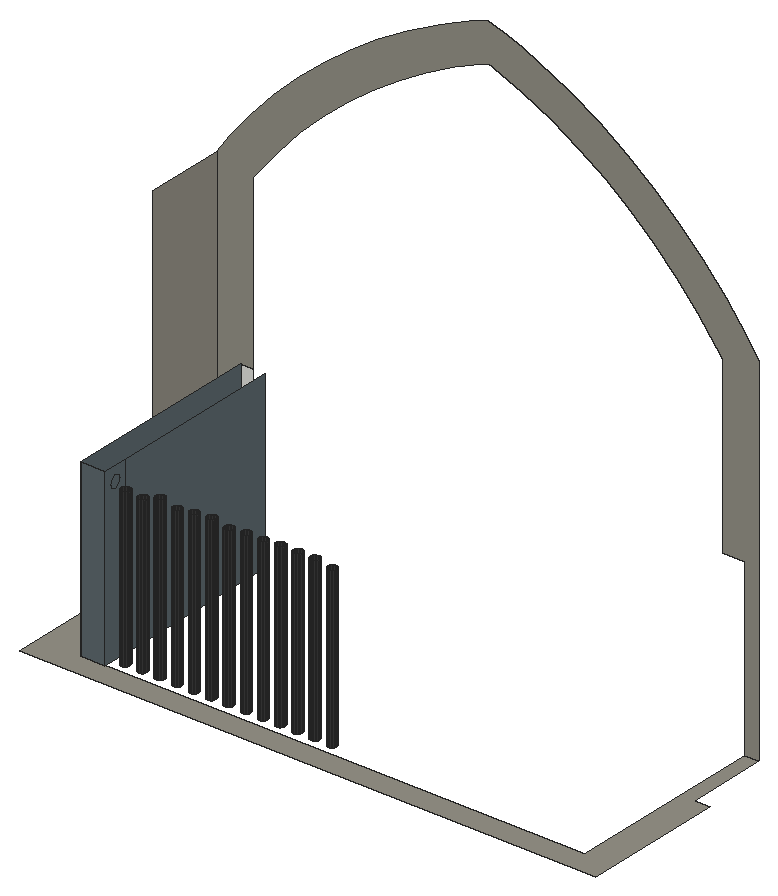
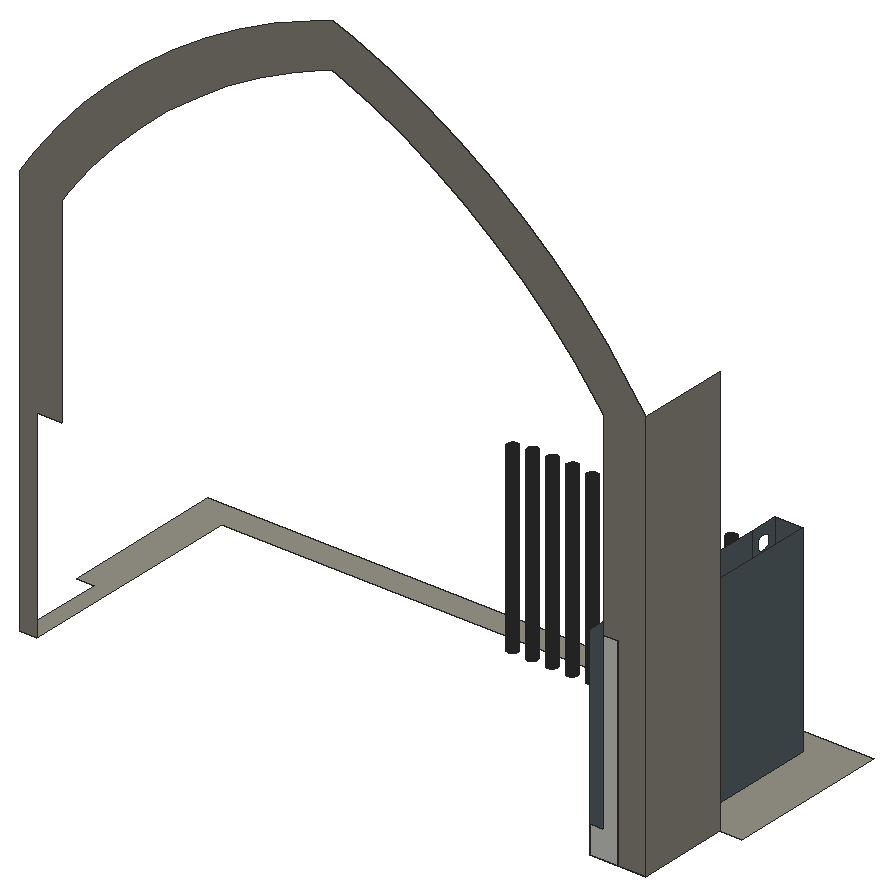
# SketchUp Ruby script. Lengths in inches.
U = 1.inch
M = Sketchup.active_model
def pt(a) = Geom::Point3d.new(a.map { |v| v * U })
def face(e, loops, mat)
  f = e.add_face(loops[0].map { |a| pt(a) })
  loops[1..].each { |l| e.add_face(l.map { |a| pt(a) }).erase! }
  f.material = f.back_material = mat if mat
  f
end
# faces: each face lists its corners as indices into pts; further lists are holes
def faces(e, pts, list, mat = nil) = list.each { |f| face(e, (f[0].is_a?(Array) ? f : [f]).map { |l| l.map { |i| pts[i] } }, mat) }
# xy, xz, yz: faces in a plane at the given z, y or x. An outline is a flat list of corners, or four numbers for a rectangle; further outlines are holes
def ring(l) = l.size == 4 ? [[l[0], l[1]], [l[2], l[1]], [l[2], l[3]], [l[0], l[3]]] : l.each_slice(2).to_a
def flat(e, list, mat, &to3) = list.each { |f| face(e, (f[0].is_a?(Array) ? f : [f]).map { |l| ring(l).map { |u, v| to3.(u, v) } }, mat) }
def xy(e, z, list, mat = nil) = flat(e, list, mat) { |x, y| [x, y, z] }
def xz(e, y, list, mat = nil) = flat(e, list, mat) { |x, z| [x, y, z] }
def yz(e, x, list, mat = nil) = flat(e, list, mat) { |y, z| [x, y, z] }
def lines(e, pts, list) = list.each { |a, b| e.add_line(pt(pts[a]), pt(pts[b])) }
# prism: a flat outline (further loops are holes) pulled along v
def prism(e, loops, v, mat = nil)
  f = face(e, loops, mat); d = Geom::Vector3d.new(v.map { |x| x * U })
  f.pushpull(f.normal.samedirection?(d) ? d.length : -d.length)
end
def box(e, o, s, mat = nil) = prism(e, [[o, [o[0] + s[0], o[1], o[2]], [o[0] + s[0], o[1] + s[1], o[2]], [o[0], o[1] + s[1], o[2]]]], [0, 0, s[2]], mat)
def at(x, y, z, deg = 0) = Geom::Transformation.translation(pt([x, y, z])) * Geom::Transformation.rotation(ORIGIN, Z_AXIS, deg.degrees)
def axes(o, x, y, z) = Geom::Transformation.new([*x, 0, *y, 0, *z, 0, *pt(o).to_a, 1])
def part(name) = M.definitions.add(name)
# library, detail: a bought-in or finely detailed component or shape, given as its bounding box
def library(name, o, s) = part(name).tap { |d| box(d.entities, o, s) }
def detail(e, o, s) = box(e.add_group.entities, o, s)
def put(e, d, t, mat = nil) = e.add_instance(d, t).tap { |i| i.material = mat if mat }
def group(e, t, mat = nil) = e.add_group.tap { |g| g.transformation = t; g.material = mat if mat }.entities
root = M.entities
M.materials.add("[Color M07]").color = [58, 58, 58]
M.materials.add("[Formica Graystone]").color = [149, 146, 135]
M.materials.add("[Formica Speckled Grey]").color = [94, 105, 111]
xy(root,557.29,[[223.35,116.47,226.66,144.04],[228.1,117.55,227.9375,117.57,227.79,117.63,227.66,117.73,227.56,117.86,227.5,118.01,227.48,118.17,227.5,118.33,227.56,118.48,227.66,118.61,227.79,118.71,227.9375,118.77,228.1,118.8,228.26,118.77,228.41,118.71,228.54,118.61,228.64,118.48,228.7,118.33,228.73,118.17,228.7,118.01,228.64,117.86,228.54,117.73,228.41,117.63,228.26,117.57],[230.48,117.55,230.3125,117.57,230.16,117.63,230.03,117.73,229.93,117.86,229.87,118.01,229.85,118.17,229.87,118.33,229.93,118.48,230.03,118.61,230.16,118.71,230.3125,118.77,230.48,118.8,230.64,118.77,230.79,118.71,230.92,118.61,231.02,118.48,231.08,118.33,231.1,118.17,231.08,118.01,231.02,117.86,230.92,117.73,230.79,117.63,230.64,117.57],[232.85,117.55,232.6875,117.57,232.54,117.63,232.41,117.73,232.31,117.86,232.25,118.01,232.23,118.17,232.25,118.33,232.31,118.48,232.41,118.61,232.54,118.71,232.6875,118.77,232.85,118.8,233.01,118.77,233.16,118.71,233.29,118.61,233.39,118.48,233.45,118.33,233.48,118.17,233.45,118.01,233.39,117.86,233.29,117.73,233.16,117.63,233.01,117.57],[235.23,117.55,235.0625,117.57,234.91,117.63,234.78,117.73,234.68,117.86,234.62,118.01,234.6,118.17,234.62,118.33,234.68,118.48,234.78,118.61,234.91,118.71,235.0625,118.77,235.23,118.8,235.39,118.77,235.54,118.71,235.67,118.61,235.77,118.48,235.83,118.33,235.85,118.17,235.83,118.01,235.77,117.86,235.67,117.73,235.54,117.63,235.39,117.57],
  [237.6,117.55,237.4375,117.57,237.29,117.63,237.16,117.73,237.06,117.86,237,118.01,236.98,118.17,237,118.33,237.06,118.48,237.16,118.61,237.29,118.71,237.4375,118.77,237.6,118.8,237.76,118.77,237.91,118.71,238.04,118.61,238.14,118.48,238.2,118.33,238.23,118.17,238.2,118.01,238.14,117.86,238.04,117.73,237.91,117.63,237.76,117.57],[239.98,117.55,239.8125,117.57,239.66,117.63,239.53,117.73,239.43,117.86,239.37,118.01,239.35,118.17,239.37,118.33,239.43,118.48,239.53,118.61,239.66,118.71,239.8125,118.77,239.98,118.8,240.14,118.77,240.29,118.71,240.42,118.61,240.52,118.48,240.58,118.33,240.6,118.17,240.58,118.01,240.52,117.86,240.42,117.73,240.29,117.63,240.14,117.57],[242.35,117.55,242.1875,117.57,242.04,117.63,241.91,117.73,241.81,117.86,241.75,118.01,241.73,118.17,241.75,118.33,241.81,118.48,241.91,118.61,242.04,118.71,242.1875,118.77,242.35,118.8,242.51,118.77,242.66,118.71,242.79,118.61,242.89,118.48,242.95,118.33,242.98,118.17,242.95,118.01,242.89,117.86,242.79,117.73,242.66,117.63,242.51,117.57],[244.73,117.55,244.5625,117.57,244.41,117.63,244.28,117.73,244.18,117.86,244.12,118.01,244.1,118.17,244.12,118.33,244.18,118.48,244.28,118.61,244.41,118.71,244.5625,118.77,244.73,118.8,244.89,118.77,245.04,118.71,245.17,118.61,245.27,118.48,245.33,118.33,245.35,118.17,245.33,118.01,245.27,117.86,245.17,117.73,245.04,117.63,244.89,117.57],[247.1,117.55,246.9375,117.57,246.79,117.63,246.66,117.73,246.56,117.86,246.5,118.01,246.48,118.17,246.5,118.33,246.56,118.48,246.66,118.61,246.79,118.71,246.9375,118.77,247.1,118.8,247.26,118.77,247.41,118.71,247.54,118.61,247.64,118.48,247.7,118.33,247.73,118.17,247.7,118.01,247.64,117.86,247.54,117.73,247.41,117.63,247.26,117.57],
  [249.48,117.55,249.3125,117.57,249.16,117.63,249.03,117.73,248.93,117.86,248.87,118.01,248.85,118.17,248.87,118.33,248.93,118.48,249.03,118.61,249.16,118.71,249.3125,118.77,249.48,118.8,249.64,118.77,249.79,118.71,249.92,118.61,250.02,118.48,250.08,118.33,250.1,118.17,250.08,118.01,250.02,117.86,249.92,117.73,249.79,117.63,249.64,117.57],[251.85,117.55,251.6875,117.57,251.54,117.63,251.41,117.73,251.31,117.86,251.25,118.01,251.23,118.17,251.25,118.33,251.31,118.48,251.41,118.61,251.54,118.71,251.6875,118.77,251.85,118.8,252.01,118.77,252.16,118.71,252.29,118.61,252.39,118.48,252.45,118.33,252.48,118.17,252.45,118.01,252.39,117.86,252.29,117.73,252.16,117.63,252.01,117.57],[254.23,117.55,254.0625,117.57,253.91,117.63,253.78,117.73,253.68,117.86,253.62,118.01,253.6,118.17,253.62,118.33,253.68,118.48,253.78,118.61,253.91,118.71,254.0625,118.77,254.23,118.8,254.39,118.77,254.54,118.71,254.67,118.61,254.77,118.48,254.83,118.33,254.85,118.17,254.83,118.01,254.77,117.86,254.67,117.73,254.54,117.63,254.39,117.57],[256.6,117.55,256.4375,117.57,256.29,117.63,256.16,117.73,256.06,117.86,256,118.01,255.98,118.17,256,118.33,256.06,118.48,256.16,118.61,256.29,118.71,256.4375,118.77,256.6,118.8,256.76,118.77,256.91,118.71,257.04,118.61,257.14,118.48,257.2,118.33,257.23,118.17,257.2,118.01,257.14,117.86,257.04,117.73,256.91,117.63,256.76,117.57]])
xy(root,557.29,[[217.39,113.35,296.83,113.35,296.83,132.97,294.7,132.97,294.7,144.04,292.74,144.04,292.74,116.47,223.35,116.47,223.35,144.04,220.02,144.04,220.02,132.97,217.39,132.97]],"[Formica Graystone]")
xz(root,116.47,[[223.35,557.29,226.66,581.29]],"[Formica Speckled Grey]")
xz(root,144.04,[[223.35,557.29,226.66,557.29,226.66,560.54,225.01,560.54,225.01,581.29,223.35,581.29]])
xz(root,144.04,[[220.02,557.29,223.35,557.29,223.35,581.29,225.01,581.29,225.01,604.82,225.75,605.875,228.5,609.35,231.45,612.66,234.59,615.78,237.91,618.71,241.4,621.4375,245.05,623.95,248.84,626.24,252.76,628.31,256.79,630.13,257.48,630.4,258.17,630.16,262.22,628.45,266.14,626.49,269.93,624.27,273.56,621.8125,277.03,619.12,280.31,616.21,283.39,613.09,286.27,609.77,288.92,606.28,289.71,605.08,289.71,581.29,292.74,581.29,292.74,557.29,294.7,557.29,294.7,606.58,293,609.17,290.15,612.92,287.06,616.49,283.75,619.84,280.22,622.97,276.5,625.86,272.59,628.5,268.52,630.88,264.31,632.99,262.125,633.92,259.96,634.83,257.4,635.71,254.87,634.75,252.55,633.7,250.5625,632.8,246.38,630.6,242.33,628.15,238.44,625.46,234.72,622.55,231.17,619.43,227.82,616.09,224.67,612.57,221.74,608.86,220.02,606.39]],"[Formica Graystone]")
yz(root,220.02,[[132.97,557.29,144.04,606.39]],"[Formica Graystone]")
yz(root,223.35,[[116.47,557.29,144.04,581.29]],"[Formica Speckled Grey]")
yz(root,226.66,[[[116.47,557.29,119.78,581.29],[118.19,578.44,117.96,578.47,117.75,578.56,117.57,578.7,117.43,578.88,117.34,579.09,117.31,579.32,117.34,579.54,117.43,579.76,117.57,579.9375,117.75,580.08,117.96,580.16,118.19,580.19,118.41,580.16,118.62,580.08,118.8,579.9375,118.94,579.76,119.03,579.54,119.06,579.32,119.03,579.09,118.94,578.88,118.8,578.7,118.62,578.56,118.41,578.47]],[119.78,557.29,144.04,581.29]],"[Formica Speckled Grey]")
p = [[227.9375,117.57,557.29],[228.1,117.55,557.29],[228.1,117.55,578.86],[227.9375,117.57,578.86],[227.9375,117.57,578.7],[228.26,117.57,557.29],
  [228.26,117.57,578.7],[228.26,117.57,578.86],[230.3125,117.57,557.29],[230.48,117.55,557.29],[230.48,117.55,578.67],[230.3125,117.57,578.67],
  [230.64,117.57,557.29],[230.64,117.57,578.67],[232.6875,117.57,557.29],[232.85,117.55,557.29],[232.85,117.55,579.54],[232.6875,117.57,579.54],
  [232.6875,117.57,578.7],[233.01,117.57,557.29],[233.01,117.57,578.7],[233.01,117.57,579.54],[235.0625,117.57,557.29],[235.23,117.55,557.29],
  [235.23,117.55,578.98],[235.0625,117.57,578.98],[235.0625,117.57,578.7],[235.39,117.57,557.29],[235.39,117.57,578.7],[235.39,117.57,578.98],
  [237.4375,117.57,557.29],[237.6,117.55,557.29],[237.6,117.55,579.32],[237.4375,117.57,579.32],[237.4375,117.57,578.7],[237.76,117.57,557.29],
  [237.76,117.57,578.7],[237.76,117.57,579.32],[239.8125,117.57,557.29],[239.98,117.55,557.29],[239.98,117.55,579.54],[239.8125,117.57,579.54],
  [239.8125,117.57,578.7],[240.14,117.57,557.29],[240.14,117.57,578.7],[240.14,117.57,579.54],[242.1875,117.57,557.29],[242.35,117.55,557.29],
  [242.35,117.55,579.09],[242.1875,117.57,579.09],[242.1875,117.57,578.7],[242.51,117.57,557.29],[242.51,117.57,578.7],[242.51,117.57,579.09],
  [244.5625,117.57,557.29],[244.73,117.55,557.29],[244.73,117.55,579.32],[244.5625,117.57,579.32],[244.5625,117.57,578.7],[244.89,117.57,557.29],
  [244.89,117.57,578.7],[244.89,117.57,579.32],[246.9375,117.57,557.29],[247.1,117.55,557.29],[247.1,117.55,579.32],[246.9375,117.57,579.32],
  [246.9375,117.57,578.7],[247.26,117.57,557.29],[247.26,117.57,578.7],[247.26,117.57,579.32],[249.3125,117.57,557.29],[249.48,117.55,557.29],
  [249.48,117.55,579.54],[249.3125,117.57,579.54],[249.3125,117.57,578.7],[249.64,117.57,557.29],[249.64,117.57,578.7],[249.64,117.57,579.54],
  [251.6875,117.57,557.29],[251.85,117.55,557.29],[251.85,117.55,579.54],[251.6875,117.57,579.54],[251.6875,117.57,578.7],[252.01,117.57,557.29],
  [252.01,117.57,578.7],[252.01,117.57,579.54],[254.0625,117.57,557.29],[254.23,117.55,557.29],[254.23,117.55,579.54],[254.0625,117.57,579.54],
  [254.0625,117.57,578.7],[254.39,117.57,557.29],[254.39,117.57,578.7],[254.39,117.57,579.54],[256.4375,117.57,557.29],[256.6,117.55,557.29],
  [256.6,117.55,579.17],[256.4375,117.57,579.17],[256.4375,117.57,578.7],[256.76,117.57,557.29],[256.76,117.57,578.7],[256.76,117.57,579.17],
  [227.66,117.73,557.29],[227.79,117.63,557.29],[227.79,117.63,578.86],[227.66,117.73,578.86],[228.41,117.63,557.29],[228.41,117.63,578.86],
  [228.54,117.73,557.29],[228.54,117.73,578.86],[230.03,117.73,557.29],[230.16,117.63,557.29],[230.16,117.63,578.67],[230.03,117.73,578.67],
  [230.79,117.63,557.29],[230.79,117.63,578.67],[230.92,117.73,557.29],[230.92,117.73,578.67],[232.41,117.73,557.29],[232.54,117.63,557.29],
  [232.54,117.63,579.54],[232.41,117.73,579.54],[233.16,117.63,557.29],[233.16,117.63,579.54],[233.29,117.73,557.29],[233.29,117.73,579.54],
  [234.78,117.73,557.29],[234.91,117.63,557.29],[234.91,117.63,578.98],[234.78,117.73,578.98],[235.54,117.63,557.29],[235.54,117.63,578.98],
  [235.67,117.73,557.29],[235.67,117.73,578.98],[237.16,117.73,557.29],[237.29,117.63,557.29],[237.29,117.63,579.32],[237.16,117.73,579.32],
  [237.91,117.63,557.29],[237.91,117.63,579.32],[238.04,117.73,557.29],[238.04,117.73,579.32],[239.53,117.73,557.29],[239.66,117.63,557.29],
  [239.66,117.63,579.54],[239.53,117.73,579.54],[240.29,117.63,557.29],[240.29,117.63,579.54],[240.42,117.73,557.29],[240.42,117.73,579.54],
  [241.91,117.73,557.29],[242.04,117.63,557.29],[242.04,117.63,579.09],[241.91,117.73,579.09],[242.66,117.63,557.29],[242.66,117.63,579.09],
  [242.79,117.73,557.29],[242.79,117.73,579.09],[244.28,117.73,557.29],[244.41,117.63,557.29],[244.41,117.63,579.32],[244.28,117.73,579.32],
  [245.04,117.63,557.29],[245.04,117.63,579.32],[245.17,117.73,557.29],[245.17,117.73,579.32],[246.66,117.73,557.29],[246.79,117.63,557.29],
  [246.79,117.63,579.32],[246.66,117.73,579.32],[247.41,117.63,557.29],[247.41,117.63,579.32],[247.54,117.73,557.29],[247.54,117.73,579.32],
  [249.03,117.73,557.29],[249.16,117.63,557.29],[249.16,117.63,579.54],[249.03,117.73,579.54],[249.79,117.63,557.29],[249.79,117.63,579.54],
  [249.92,117.73,557.29],[249.92,117.73,579.54],[251.41,117.73,557.29],[251.54,117.63,557.29],[251.54,117.63,579.54],[251.41,117.73,579.54],
  [252.16,117.63,557.29],[252.16,117.63,579.54],[252.29,117.73,557.29],[252.29,117.73,579.54],[253.78,117.73,557.29],[253.91,117.63,557.29],
  [253.91,117.63,579.54],[253.78,117.73,579.54],[254.54,117.63,557.29],[254.54,117.63,579.54],[254.67,117.73,557.29],[254.67,117.73,579.54],
  [256.16,117.73,557.29],[256.29,117.63,557.29],[256.29,117.63,579.17],[256.16,117.73,579.17],[256.91,117.63,557.29],[256.91,117.63,579.17],
  [257.04,117.73,557.29],[257.04,117.73,579.17],[227.56,117.86,557.29],[227.56,117.86,578.86],[228.64,117.86,557.29],[228.64,117.86,578.86],
  [229.93,117.86,557.29],[229.93,117.86,578.67],[231.02,117.86,557.29],[231.02,117.86,578.67],[232.31,117.86,557.29],[232.31,117.86,579.54],
  [233.39,117.86,557.29],[233.39,117.86,579.54],[234.68,117.86,557.29],[234.68,117.86,578.98],[235.77,117.86,557.29],[235.77,117.86,578.98],
  [237.06,117.86,557.29],[237.06,117.86,579.32],[238.14,117.86,557.29],[238.14,117.86,579.32],[239.43,117.86,557.29],[239.43,117.86,579.54],
  [240.52,117.86,557.29],[240.52,117.86,579.54],[241.81,117.86,557.29],[241.81,117.86,579.09],[242.89,117.86,557.29],[242.89,117.86,579.09],
  [244.18,117.86,557.29],[244.18,117.86,579.32],[245.27,117.86,557.29],[245.27,117.86,579.32],[246.56,117.86,557.29],[246.56,117.86,579.32],
  [247.64,117.86,557.29],[247.64,117.86,579.32],[248.93,117.86,557.29],[248.93,117.86,579.54],[250.02,117.86,557.29],[250.02,117.86,579.54],
  [251.31,117.86,557.29],[251.31,117.86,579.54],[252.39,117.86,557.29],[252.39,117.86,579.54],[253.68,117.86,557.29],[253.68,117.86,579.54],
  [254.77,117.86,557.29],[254.77,117.86,579.54],[256.06,117.86,557.29],[256.06,117.86,579.17],[257.14,117.86,557.29],[257.14,117.86,579.17],
  [227.5,118.01,557.29],[227.5,118.01,578.86],[228.7,118.01,557.29],[228.7,118.01,578.86],[229.87,118.01,557.29],[229.87,118.01,578.67],
  [231.08,118.01,557.29],[231.08,118.01,578.67],[232.25,118.01,557.29],[232.25,118.01,579.54],[233.45,118.01,557.29],[233.45,118.01,579.54],
  [234.62,118.01,557.29],[234.62,118.01,578.98],[235.83,118.01,557.29],[235.83,118.01,578.98],[237,118.01,557.29],[237,118.01,579.32],
  [238.2,118.01,557.29],[238.2,118.01,579.32],[239.37,118.01,557.29],[239.37,118.01,579.54],[240.58,118.01,557.29],[240.58,118.01,579.54],
  [241.75,118.01,557.29],[241.75,118.01,579.09],[242.95,118.01,557.29],[242.95,118.01,579.09],[244.12,118.01,557.29],[244.12,118.01,579.32],
  [245.33,118.01,557.29],[245.33,118.01,579.32],[246.5,118.01,557.29],[246.5,118.01,579.32],[247.7,118.01,557.29],[247.7,118.01,579.32],
  [248.87,118.01,557.29],[248.87,118.01,579.54],[250.08,118.01,557.29],[250.08,118.01,579.54],[251.25,118.01,557.29],[251.25,118.01,579.54],
  [252.45,118.01,557.29],[252.45,118.01,579.54],[253.62,118.01,557.29],[253.62,118.01,579.54],[254.83,118.01,557.29],[254.83,118.01,579.54],
  [256,118.01,557.29],[256,118.01,579.17],[257.2,118.01,557.29],[257.2,118.01,579.17],[227.48,118.17,557.29],[227.48,118.17,578.86],
  [228.73,118.17,557.29],[228.73,118.17,578.86],[229.85,118.17,557.29],[229.85,118.17,578.67],[231.1,118.17,557.29],[231.1,118.17,578.67],
  [232.23,118.17,557.29],[232.23,118.17,579.54],[233.48,118.17,557.29],[233.48,118.17,579.54],[234.6,118.17,557.29],[234.6,118.17,578.98],
  [235.85,118.17,557.29],[235.85,118.17,578.98],[236.98,118.17,557.29],[236.98,118.17,579.32],[238.23,118.17,557.29],[238.23,118.17,579.32],
  [239.35,118.17,557.29],[239.35,118.17,579.54],[240.6,118.17,557.29],[240.6,118.17,579.54],[241.73,118.17,557.29],[241.73,118.17,579.09],
  [242.98,118.17,557.29],[242.98,118.17,579.09],[244.1,118.17,557.29],[244.1,118.17,579.32],[245.35,118.17,557.29],[245.35,118.17,579.32],
  [246.48,118.17,557.29],[246.48,118.17,579.32],[247.73,118.17,557.29],[247.73,118.17,579.32],[248.85,118.17,557.29],[248.85,118.17,579.54],
  [250.1,118.17,557.29],[250.1,118.17,579.54],[251.23,118.17,557.29],[251.23,118.17,579.54],[252.48,118.17,557.29],[252.48,118.17,579.54],
  [253.6,118.17,557.29],[253.6,118.17,579.54],[254.85,118.17,557.29],[254.85,118.17,579.54],[255.98,118.17,557.29],[255.98,118.17,579.17],
  [257.23,118.17,557.29],[257.23,118.17,579.17],[227.5,118.33,557.29],[227.5,118.33,578.86],[228.7,118.33,557.29],[228.7,118.33,578.86],
  [229.87,118.33,557.29],[229.87,118.33,578.67],[231.08,118.33,557.29],[231.08,118.33,578.67],[232.25,118.33,557.29],[232.25,118.33,579.54],
  [233.45,118.33,557.29],[233.45,118.33,579.54],[234.62,118.33,557.29],[234.62,118.33,578.98],[235.83,118.33,557.29],[235.83,118.33,578.98],
  [237,118.33,557.29],[237,118.33,579.32],[238.2,118.33,557.29],[238.2,118.33,579.32],[239.37,118.33,557.29],[239.37,118.33,579.54],
  [240.58,118.33,557.29],[240.58,118.33,579.54],[241.75,118.33,557.29],[241.75,118.33,579.09],[242.95,118.33,557.29],[242.95,118.33,579.09],
  [244.12,118.33,557.29],[244.12,118.33,579.32],[245.33,118.33,557.29],[245.33,118.33,579.32],[246.5,118.33,557.29],[246.5,118.33,579.32],
  [247.7,118.33,557.29],[247.7,118.33,579.32],[248.87,118.33,557.29],[248.87,118.33,579.54],[250.08,118.33,557.29],[250.08,118.33,579.54],
  [251.25,118.33,557.29],[251.25,118.33,579.54],[252.45,118.33,557.29],[252.45,118.33,579.54],[253.62,118.33,557.29],[253.62,118.33,579.54],
  [254.83,118.33,557.29],[254.83,118.33,579.54],[256,118.33,557.29],[256,118.33,579.17],[257.2,118.33,557.29],[257.2,118.33,579.17],
  [227.56,118.48,557.29],[227.56,118.48,578.86],[228.64,118.48,557.29],[228.64,118.48,578.86],[229.93,118.48,557.29],[229.93,118.48,578.67],
  [231.02,118.48,557.29],[231.02,118.48,578.67],[232.31,118.48,557.29],[232.31,118.48,579.54],[233.39,118.48,557.29],[233.39,118.48,579.54],
  [234.68,118.48,557.29],[234.68,118.48,578.98],[235.77,118.48,557.29],[235.77,118.48,578.98],[237.06,118.48,557.29],[237.06,118.48,579.32],
  [238.14,118.48,557.29],[238.14,118.48,579.32],[239.43,118.48,557.29],[239.43,118.48,579.54],[240.52,118.48,557.29],[240.52,118.48,579.54],
  [241.81,118.48,557.29],[241.81,118.48,579.09],[242.89,118.48,557.29],[242.89,118.48,579.09],[244.18,118.48,557.29],[244.18,118.48,579.32],
  [245.27,118.48,557.29],[245.27,118.48,579.32],[246.56,118.48,557.29],[246.56,118.48,579.32],[247.64,118.48,557.29],[247.64,118.48,579.32],
  [248.93,118.48,557.29],[248.93,118.48,579.54],[250.02,118.48,557.29],[250.02,118.48,579.54],[251.31,118.48,557.29],[251.31,118.48,579.54],
  [252.39,118.48,557.29],[252.39,118.48,579.54],[253.68,118.48,557.29],[253.68,118.48,579.54],[254.77,118.48,557.29],[254.77,118.48,579.54],
  [256.06,118.48,557.29],[256.06,118.48,579.17],[257.14,118.48,557.29],[257.14,118.48,579.17],[227.66,118.61,557.29],[227.66,118.61,578.86],
  [228.54,118.61,557.29],[228.54,118.61,578.86],[230.03,118.61,557.29],[230.03,118.61,578.67],[230.92,118.61,557.29],[230.92,118.61,578.67],
  [232.41,118.61,557.29],[232.41,118.61,579.54],[233.29,118.61,557.29],[233.29,118.61,579.54],[234.78,118.61,557.29],[234.78,118.61,578.98],
  [235.67,118.61,557.29],[235.67,118.61,578.98],[237.16,118.61,557.29],[237.16,118.61,579.32],[238.04,118.61,557.29],[238.04,118.61,579.32],
  [239.53,118.61,557.29],[239.53,118.61,579.54],[240.42,118.61,557.29],[240.42,118.61,579.54],[241.91,118.61,557.29],[241.91,118.61,579.09],
  [242.79,118.61,557.29],[242.79,118.61,579.09],[244.28,118.61,557.29],[244.28,118.61,579.32],[245.17,118.61,557.29],[245.17,118.61,579.32],
  [246.66,118.61,557.29],[246.66,118.61,579.32],[247.54,118.61,557.29],[247.54,118.61,579.32],[249.03,118.61,557.29],[249.03,118.61,579.54],
  [249.92,118.61,557.29],[249.92,118.61,579.54],[251.41,118.61,557.29],[251.41,118.61,579.54],[252.29,118.61,557.29],[252.29,118.61,579.54],
  [253.78,118.61,557.29],[253.78,118.61,579.54],[254.67,118.61,557.29],[254.67,118.61,579.54],[256.16,118.61,557.29],[256.16,118.61,579.17],
  [257.04,118.61,557.29],[257.04,118.61,579.17],[227.79,118.71,557.29],[227.79,118.71,578.86],[228.41,118.71,557.29],[228.41,118.71,578.86],
  [230.16,118.71,557.29],[230.16,118.71,578.67],[230.79,118.71,557.29],[230.79,118.71,578.67],[232.54,118.71,557.29],[232.54,118.71,579.54],
  [233.16,118.71,557.29],[233.16,118.71,579.54],[234.91,118.71,557.29],[234.91,118.71,578.98],[235.54,118.71,557.29],[235.54,118.71,578.98],
  [237.29,118.71,557.29],[237.29,118.71,579.32],[237.91,118.71,557.29],[237.91,118.71,579.32],[239.66,118.71,557.29],[239.66,118.71,579.54],
  [240.29,118.71,557.29],[240.29,118.71,579.54],[242.04,118.71,557.29],[242.04,118.71,579.09],[242.66,118.71,557.29],[242.66,118.71,579.09],
  [244.41,118.71,557.29],[244.41,118.71,579.32],[245.04,118.71,557.29],[245.04,118.71,579.32],[246.79,118.71,557.29],[246.79,118.71,579.32],
  [247.41,118.71,557.29],[247.41,118.71,579.32],[249.16,118.71,557.29],[249.16,118.71,579.54],[249.79,118.71,557.29],[249.79,118.71,579.54],
  [251.54,118.71,557.29],[251.54,118.71,579.54],[252.16,118.71,557.29],[252.16,118.71,579.54],[253.91,118.71,557.29],[253.91,118.71,579.54],
  [254.54,118.71,557.29],[254.54,118.71,579.54],[256.29,118.71,557.29],[256.29,118.71,579.17],[256.91,118.71,557.29],[256.91,118.71,579.17],
  [227.9375,118.77,557.29],[227.9375,118.77,578.86],[228.26,118.77,557.29],[228.26,118.77,578.86],[230.3125,118.77,557.29],[230.3125,118.77,578.67],
  [230.64,118.77,557.29],[230.64,118.77,578.67],[232.6875,118.77,557.29],[232.6875,118.77,579.54],[233.01,118.77,557.29],[233.01,118.77,579.54],
  [235.0625,118.77,557.29],[235.0625,118.77,578.98],[235.39,118.77,557.29],[235.39,118.77,578.98],[237.4375,118.77,557.29],[237.4375,118.77,579.32],
  [237.76,118.77,557.29],[237.76,118.77,579.32],[239.8125,118.77,557.29],[239.8125,118.77,579.54],[240.14,118.77,557.29],[240.14,118.77,579.54],
  [242.1875,118.77,557.29],[242.1875,118.77,579.09],[242.51,118.77,557.29],[242.51,118.77,579.09],[244.5625,118.77,557.29],[244.5625,118.77,579.32],
  [244.89,118.77,557.29],[244.89,118.77,579.32],[246.9375,118.77,557.29],[246.9375,118.77,579.32],[247.26,118.77,557.29],[247.26,118.77,579.32],
  [249.3125,118.77,557.29],[249.3125,118.77,579.54],[249.64,118.77,557.29],[249.64,118.77,579.54],[251.6875,118.77,557.29],[251.6875,118.77,579.54],
  [252.01,118.77,557.29],[252.01,118.77,579.54],[254.0625,118.77,557.29],[254.0625,118.77,579.54],[254.39,118.77,557.29],[254.39,118.77,579.54],
  [256.4375,118.77,557.29],[256.4375,118.77,579.17],[256.76,118.77,557.29],[256.76,118.77,579.17],[228.1,118.8,557.29],[228.1,118.8,578.86],
  [230.48,118.8,557.29],[230.48,118.8,578.67],[232.85,118.8,557.29],[232.85,118.8,579.54],[235.23,118.8,557.29],[235.23,118.8,578.98],
  [237.6,118.8,557.29],[237.6,118.8,579.32],[239.98,118.8,557.29],[239.98,118.8,579.54],[242.35,118.8,557.29],[242.35,118.8,579.09],
  [244.73,118.8,557.29],[244.73,118.8,579.32],[247.1,118.8,557.29],[247.1,118.8,579.32],[249.48,118.8,557.29],[249.48,118.8,579.54],
  [251.85,118.8,557.29],[251.85,118.8,579.54],[254.23,118.8,557.29],[254.23,118.8,579.54],[256.6,118.8,557.29],[256.6,118.8,579.17]]
faces(root,p,[[0,1,2,3,4],[1,5,6,7,2],[8,9,10,11],[9,12,13,10],[14,15,16,17,18],[15,19,20,21,16],[22,23,24,25,26],[23,27,28,29,24],
  [30,31,32,33,34],[31,35,36,37,32],[38,39,40,41,42],[39,43,44,45,40],[46,47,48,49,50],[47,51,52,53,48],[54,55,56,57,58],[55,59,60,61,56],
  [62,63,64,65,66],[63,67,68,69,64],[70,71,72,73,74],[71,75,76,77,72],[78,79,80,81,82],[79,83,84,85,80],[86,87,88,89,90],[87,91,92,93,88],
  [94,95,96,97,98],[95,99,100,101,96],[102,103,104,105],[103,0,4,3,104],[5,106,107,7,6],[106,108,109,107],[110,111,112,113],[111,8,11,112],
  [12,114,115,13],[114,116,117,115],[118,119,120,121],[119,14,18,17,120],[19,122,123,21,20],[122,124,125,123],[126,127,128,129],[127,22,26,25,128],
  [27,130,131,29,28],[130,132,133,131],[134,135,136,137],[135,30,34,33,136],[35,138,139,37,36],[138,140,141,139],[142,143,144,145],[143,38,42,41,144],
  [43,146,147,45,44],[146,148,149,147],[150,151,152,153],[151,46,50,49,152],[51,154,155,53,52],[154,156,157,155],[158,159,160,161],[159,54,58,57,160],
  [59,162,163,61,60],[162,164,165,163],[166,167,168,169],[167,62,66,65,168],[67,170,171,69,68],[170,172,173,171],[174,175,176,177],[175,70,74,73,176],
  [75,178,179,77,76],[178,180,181,179],[182,183,184,185],[183,78,82,81,184],[83,186,187,85,84],[186,188,189,187],[190,191,192,193],[191,86,90,89,192],
  [91,194,195,93,92],[194,196,197,195],[198,199,200,201],[199,94,98,97,200],[99,202,203,101,100],[202,204,205,203],[206,102,105,207],[108,208,209,109],
  [210,110,113,211],[116,212,213,117],[214,118,121,215],[124,216,217,125],[218,126,129,219],[132,220,221,133],[222,134,137,223],[140,224,225,141],
  [226,142,145,227],[148,228,229,149],[230,150,153,231],[156,232,233,157],[234,158,161,235],[164,236,237,165],[238,166,169,239],[172,240,241,173],
  [242,174,177,243],[180,244,245,181],[246,182,185,247],[188,248,249,189],[250,190,193,251],[196,252,253,197],[254,198,201,255],[204,256,257,205],
  [258,206,207,259],[208,260,261,209],[262,210,211,263],[212,264,265,213],[266,214,215,267],[216,268,269,217],[270,218,219,271],[220,272,273,221],
  [274,222,223,275],[224,276,277,225],[278,226,227,279],[228,280,281,229],[282,230,231,283],[232,284,285,233],[286,234,235,287],[236,288,289,237],
  [290,238,239,291],[240,292,293,241],[294,242,243,295],[244,296,297,245],[298,246,247,299],[248,300,301,249],[302,250,251,303],[252,304,305,253],
  [306,254,255,307],[256,308,309,257],[310,258,259,311],[260,312,313,261],[314,262,263,315],[264,316,317,265],[318,266,267,319],[268,320,321,269],
  [322,270,271,323],[272,324,325,273],[326,274,275,327],[276,328,329,277],[330,278,279,331],[280,332,333,281],[334,282,283,335],[284,336,337,285],
  [338,286,287,339],[288,340,341,289],[342,290,291,343],[292,344,345,293],[346,294,295,347],[296,348,349,297],[350,298,299,351],[300,352,353,301],
  [354,302,303,355],[304,356,357,305],[358,306,307,359],[308,360,361,309],[362,310,311,363],[312,364,365,313],[366,314,315,367],[316,368,369,317],
  [370,318,319,371],[320,372,373,321],[374,322,323,375],[324,376,377,325],[378,326,327,379],[328,380,381,329],[382,330,331,383],[332,384,385,333],
  [386,334,335,387],[336,388,389,337],[390,338,339,391],[340,392,393,341],[394,342,343,395],[344,396,397,345],[398,346,347,399],[348,400,401,349],
  [402,350,351,403],[352,404,405,353],[406,354,355,407],[356,408,409,357],[410,358,359,411],[360,412,413,361],[414,362,363,415],[364,416,417,365],
  [418,366,367,419],[368,420,421,369],[422,370,371,423],[372,424,425,373],[426,374,375,427],[376,428,429,377],[430,378,379,431],[380,432,433,381],
  [434,382,383,435],[384,436,437,385],[438,386,387,439],[388,440,441,389],[442,390,391,443],[392,444,445,393],[446,394,395,447],[396,448,449,397],
  [450,398,399,451],[400,452,453,401],[454,402,403,455],[404,456,457,405],[458,406,407,459],[408,460,461,409],[462,410,411,463],[412,464,465,413],
  [466,414,415,467],[416,468,469,417],[470,418,419,471],[420,472,473,421],[474,422,423,475],[424,476,477,425],[478,426,427,479],[428,480,481,429],
  [482,430,431,483],[432,484,485,433],[486,434,435,487],[436,488,489,437],[490,438,439,491],[440,492,493,441],[494,442,443,495],[444,496,497,445],
  [498,446,447,499],[448,500,501,449],[502,450,451,503],[452,504,505,453],[506,454,455,507],[456,508,509,457],[510,458,459,511],[460,512,513,461],
  [514,462,463,515],[464,516,517,465],[518,466,467,519],[468,520,521,469],[522,470,471,523],[472,524,525,473],[526,474,475,527],[476,528,529,477],
  [530,478,479,531],[480,532,533,481],[534,482,483,535],[484,536,537,485],[538,486,487,539],[488,540,541,489],[542,490,491,543],[492,544,545,493],
  [546,494,495,547],[496,548,549,497],[550,498,499,551],[500,552,553,501],[554,502,503,555],[504,556,557,505],[558,506,507,559],[508,560,561,509],
  [562,510,511,563],[512,564,565,513],[566,514,515,567],[516,568,569,517],[570,518,519,571],[520,572,573,521],[574,522,523,575],[524,576,577,525],
  [578,526,527,579],[528,580,581,529],[582,530,531,583],[532,584,585,533],[586,534,535,587],[536,588,589,537],[590,538,539,591],[540,592,593,541],
  [594,542,543,595],[544,596,597,545],[598,546,547,599],[548,600,601,549],[602,550,551,603],[552,604,605,553],[606,554,555,607],[556,608,609,557],
  [610,558,559,611],[560,612,613,561],[614,562,563,615],[564,616,617,565],[618,566,567,619],[568,620,621,569],[622,570,571,623],[572,622,623,573],
  [624,574,575,625],[576,624,625,577],[626,578,579,627],[580,626,627,581],[628,582,583,629],[584,628,629,585],[630,586,587,631],[588,630,631,589],
  [632,590,591,633],[592,632,633,593],[634,594,595,635],[596,634,635,597],[636,598,599,637],[600,636,637,601],[638,602,603,639],[604,638,639,605],
  [640,606,607,641],[608,640,641,609],[642,610,611,643],[612,642,643,613],[644,614,615,645],[616,644,645,617],[646,618,619,647],[620,646,647,621]],"[Color M07]")
